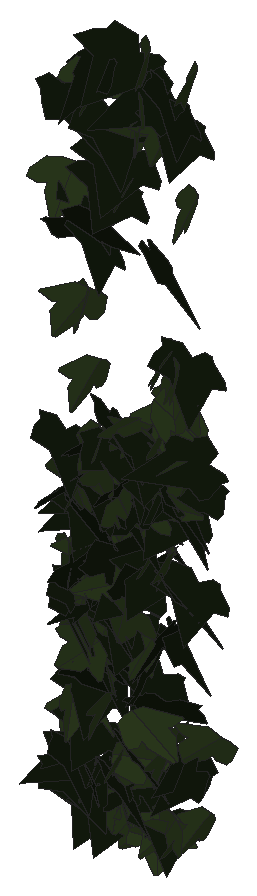
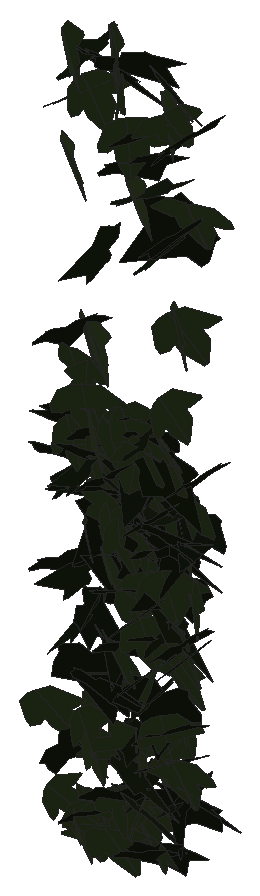
# SketchUp Ruby script. Lengths in inches.
U = 1.inch
M = Sketchup.active_model
def pt(a) = Geom::Point3d.new(a.map { |v| v * U })
def face(e, loops, mat)
  f = e.add_face(loops[0].map { |a| pt(a) })
  loops[1..].each { |l| e.add_face(l.map { |a| pt(a) }).erase! }
  f.material = f.back_material = mat if mat
  f
end
# faces: each face lists its corners as indices into pts; further lists are holes
def faces(e, pts, list, mat = nil) = list.each { |f| face(e, (f[0].is_a?(Array) ? f : [f]).map { |l| l.map { |i| pts[i] } }, mat) }
# xy, xz, yz: faces in a plane at the given z, y or x. An outline is a flat list of corners, or four numbers for a rectangle; further outlines are holes
def ring(l) = l.size == 4 ? [[l[0], l[1]], [l[2], l[1]], [l[2], l[3]], [l[0], l[3]]] : l.each_slice(2).to_a
def flat(e, list, mat, &to3) = list.each { |f| face(e, (f[0].is_a?(Array) ? f : [f]).map { |l| ring(l).map { |u, v| to3.(u, v) } }, mat) }
def xy(e, z, list, mat = nil) = flat(e, list, mat) { |x, y| [x, y, z] }
def xz(e, y, list, mat = nil) = flat(e, list, mat) { |x, z| [x, y, z] }
def yz(e, x, list, mat = nil) = flat(e, list, mat) { |y, z| [x, y, z] }
def lines(e, pts, list) = list.each { |a, b| e.add_line(pt(pts[a]), pt(pts[b])) }
# prism: a flat outline (further loops are holes) pulled along v
def prism(e, loops, v, mat = nil)
  f = face(e, loops, mat); d = Geom::Vector3d.new(v.map { |x| x * U })
  f.pushpull(f.normal.samedirection?(d) ? d.length : -d.length)
end
def box(e, o, s, mat = nil) = prism(e, [[o, [o[0] + s[0], o[1], o[2]], [o[0] + s[0], o[1] + s[1], o[2]], [o[0], o[1] + s[1], o[2]]]], [0, 0, s[2]], mat)
def at(x, y, z, deg = 0) = Geom::Transformation.translation(pt([x, y, z])) * Geom::Transformation.rotation(ORIGIN, Z_AXIS, deg.degrees)
def axes(o, x, y, z) = Geom::Transformation.new([*x, 0, *y, 0, *z, 0, *pt(o).to_a, 1])
def part(name) = M.definitions.add(name)
# library, detail: a bought-in or finely detailed component or shape, given as its bounding box
def library(name, o, s) = part(name).tap { |d| box(d.entities, o, s) }
def detail(e, o, s) = box(e.add_group.entities, o, s)
def put(e, d, t, mat = nil) = e.add_instance(d, t).tap { |i| i.material = mat if mat }
def group(e, t, mat = nil) = e.add_group.tap { |g| g.transformation = t; g.material = mat if mat }.entities
root = M.entities
M.materials.add("1026 AP 7946 SUNNY SIDE UP").color = [254, 231, 186]
M.materials.add("efeu1").color = [18, 25, 13]
M.materials.add("efeu2").color = [43, 57, 29]
c1 = part("ivyleaf_9")
p = [[1.54,2.16,1.25],[1.36,2.04,1.19],[-0.21,0.99,0.68],[-0.71,1.11,0.82],[-0.85,0.86,0.67],[-0.8,0.17,0.21],
  [-0.9,-0.01,0.1],[-0.67,-0.16,-0.02],[-0.08,-0.08,-0.05],[-0.03,-0.6,-0.4],[0.65,-0.88,-0.66],[0.83,-0.6,-0.49],
  [1.29,-0.42,-0.43],[1.8125,-0.07,-0.26],[1.21,0.44,0.15]]
faces(c1.entities,p,[[0,1,2,3,4,5,6,7,8,9,10,11,12,13,14]],"efeu1")
c2 = part("ivyleaf_10")
p = [[0,0.5,-0.03],[-0.0625,2.02,-0.43],[-0.19,2.01,-0.46],[-0.54,1.05,-0.29],[-0.52,0.625,-0.18],[-0.83,0.76,-0.28],
  [-1.16,0.64,-0.33],[-1.15,0.33,-0.24],[-0.77,-0.39,0.02],[-0.3,-0.51,0.16],[0.04,-0.48,0.23],[-0.02,2.01,-0.4375],
  [-0.06,2.01,-0.43],[0.04,-0.49,0.23],[0.67,-0.49,0.14],[1.38,0.36,-0.2],[1.375,0.51,-0.24],[0.81,0.65,-0.19],
  [0.62,0.59,-0.15],[0.6,1.09,-0.28],[0.5,1.23,-0.31]]
faces(c2.entities,p,[[0,1,2,3,4,5,6,7,8,9,10],[11,12,0,13,14,15,16,17,18,19,20]],"efeu2")
put(root,c1,axes([116.8,212.3,272.73],[0.11017,0.25618,0.13801],[0.05388,0.128,-0.27286],[-0.45031,0.07799,0.00112]),"1026 AP 7946 SUNNY SIDE UP")
put(root,c2,axes([116.82,212.65,272.72],[0.1225,-0.25561,-0.10606],[-0.04117,0.09812,-0.27469],[0.43048,0.08212,0.00391]),"1026 AP 7946 SUNNY SIDE UP")
put(root,c2,axes([116.8,212.47,271.73],[0.22805,-0.21005,-0.12772],[-0.0326,0.13175,-0.25665],[0.38118,0.13693,0.05446]),"1026 AP 7946 SUNNY SIDE UP")
put(root,c2,axes([116.78,212.79,269.29],[0.40893,0.02168,-0.05836],[-0.09133,0.01527,-0.268],[-0.02811,0.26575,0.02173]),"1026 AP 7946 SUNNY SIDE UP")
put(root,c1,axes([117,212.56,268.79],[-0.4104,0.01771,0.02308],[-0.03858,-0.03545,-0.26702],[-0.02274,-0.25954,0.0365]),"1026 AP 7946 SUNNY SIDE UP")
put(root,c1,axes([116.67,212.59,273.41],[-0.02183,-0.28584,0.04041],[-0.0034,-0.04079,-0.29506],[0.45401,-0.01405,-0.00027]),"1026 AP 7946 SUNNY SIDE UP")
put(root,c2,axes([116.76,212.55,277.26],[0.46657,0.05221,-0.03464],[-0.04289,-0.03946,-0.30864],[-0.088,0.29604,-0.03322]),"1026 AP 7946 SUNNY SIDE UP")
put(root,c1,axes([116.67,212.79,270.91],[0.04526,-0.27109,0.02421],[-0.00744,-0.02567,-0.28089],[0.42801,0.02822,-0.00744]),"1026 AP 7946 SUNNY SIDE UP")
put(root,c2,axes([117.09,212.45,270.9],[-0.21954,0.13083,0.21379],[-0.33102,0.05714,-0.18334],[-0.19614,-0.24288,0.07012]),"1026 AP 7946 SUNNY SIDE UP")
put(root,c1,axes([116.64,212.62,278.45],[0.13508,-0.28326,-0.10763],[-0.00728,0.10571,-0.30325],[0.4738,0.08238,0.02603]),"1026 AP 7946 SUNNY SIDE UP")
put(root,c1,axes([116.72,212.81,271.12],[-0.00572,-0.27971,-0.00531],[-0.00211,0.00359,-0.28815],[0.43984,-0.00362,-0.00145]),"1026 AP 7946 SUNNY SIDE UP")
put(root,c2,axes([116.86,212.55,272.92],[-0.43647,0.05098,-0.02968],[0.03875,-0.02645,-0.29006],[-0.08377,-0.27784,0.02048]),"1026 AP 7946 SUNNY SIDE UP")
put(root,c2,axes([117,212.54,275.53],[-0.23482,-0.21491,0.16004],[-0.06896,-0.15721,-0.26631],[0.41237,-0.14867,0.0466]),"1026 AP 7946 SUNNY SIDE UP")
put(root,c2,axes([116.85,212.55,269.61],[0.06416,0.22553,-0.1485],[-0.02434,-0.14488,-0.23678],[-0.42126,0.04272,-0.00894]),"1026 AP 7946 SUNNY SIDE UP")
put(root,c1,axes([117.13,212.78,272.46],[-0.43068,0.05972,0.00846],[-0.01834,-0.01663,-0.28825],[-0.09292,-0.27351,0.0177]),"1026 AP 7946 SUNNY SIDE UP")
put(root,c2,axes([116.92,212.84,278.66],[0.26812,0.21109,-0.15435],[-0.11163,-0.13588,-0.27902],[-0.39255,0.18281,-0.02608]),"1026 AP 7946 SUNNY SIDE UP")
put(root,c2,axes([116.98,212.84,269.85],[-0.24545,-0.21557,0.05732],[0.01059,-0.07394,-0.27018],[0.3504,-0.14877,0.04831]),"1026 AP 7946 SUNNY SIDE UP")
put(root,c1,axes([117.0625,212.48,268.72],[0.17257,-0.01247,-0.25671],[-0.38054,0.06053,-0.11261],[0.0949,0.2654,0.01526]),"1026 AP 7946 SUNNY SIDE UP")
put(root,c1,axes([116.78,212.87,277.03],[0.05506,-0.29844,-0.03977],[-0.00588,0.03672,-0.30934],[0.47281,0.03521,0.00078]),"1026 AP 7946 SUNNY SIDE UP")
put(root,c2,axes([117.01,212.73,274.4],[-0.10231,-0.25018,0.14867],[0.02311,-0.15203,-0.263],[0.45468,-0.04857,0.04682]),"1026 AP 7946 SUNNY SIDE UP")
put(root,c1,axes([117.21,212.875,272.64],[-0.42962,0.00079,0.06113],[-0.09186,-0.05248,-0.27674],[0.01631,-0.27462,0.0514]),"1026 AP 7946 SUNNY SIDE UP")
put(root,c1,axes([117.16,212.625,273.46],[-0.09378,0.24669,-0.12343],[0.00527,-0.12338,-0.26109],[-0.43217,-0.05504,0.0236]),"1026 AP 7946 SUNNY SIDE UP")
put(root,c2,axes([117.07,212.69,271.83],[-0.31265,-0.18899,0.06939],[-0.00898,-0.0909,-0.27627],[0.31592,-0.18962,0.06081]),"1026 AP 7946 SUNNY SIDE UP")
put(root,c1,axes([116.83,212.58,268.75],[0.03707,-0.26163,0.10666],[0.04398,-0.10269,-0.27063],[0.44111,0.03223,0.01802]),"1026 AP 7946 SUNNY SIDE UP")
put(root,c1,axes([116.97,212.85,269.76],[-0.16699,-0.2477,0.03137],[0.01363,-0.03826,-0.27687],[0.39246,-0.10407,0.02296]),"1026 AP 7946 SUNNY SIDE UP")
put(root,c1,axes([117.05,212.87,268.1],[-0.32164,-0.15592,-0.03351],[0.05965,0.00226,-0.26407],[0.24295,-0.20697,0.02047]),"1026 AP 7946 SUNNY SIDE UP")
put(root,c1,axes([117.22,212.49,271.24],[-0.26058,0.22191,-0.0552],[0.03561,-0.05146,-0.28534],[-0.35767,-0.1668,0.01181]),"1026 AP 7946 SUNNY SIDE UP")
put(root,c2,axes([117.05,212.48,275.55],[0.20251,-0.25936,-0.06125],[-0.0095,0.06156,-0.29713],[0.41777,0.12712,0.02294]),"1026 AP 7946 SUNNY SIDE UP")
put(root,c1,axes([117.03,212.82,272.38],[-0.2351,-0.23696,0.04936],[0.01399,-0.06324,-0.28596],[0.3803,-0.14416,0.04103]),"1026 AP 7946 SUNNY SIDE UP")
put(root,c2,axes([117.11,212.61,278.68],[0.12774,-0.27589,-0.1203],[-0.02856,0.11461,-0.29527],[0.46925,0.08208,0.01478]),"1026 AP 7946 SUNNY SIDE UP")
put(root,c1,axes([117.03,212.48,272.4],[0.36695,-0.02613,-0.15604],[-0.24041,-0.01388,-0.24053],[0.0225,0.27779,-0.02505]),"1026 AP 7946 SUNNY SIDE UP")
put(root,c2,axes([117.19,212.41,270.54],[0.34925,-0.1127,-0.14779],[-0.20274,0.0615,-0.25621],[0.20182,0.2568,-0.00163]),"1026 AP 7946 SUNNY SIDE UP")
put(root,c1,axes([117.02,212.3,271.74],[-0.04223,0.0915,-0.28021],[-0.09387,0.26596,0.09962],[0.44216,0.0652,-0.00562]),"1026 AP 7946 SUNNY SIDE UP")
put(root,c1,axes([116.91,212.49,268.64],[-0.18108,-0.1399,-0.21192],[0.23475,0.14137,-0.18504],[0.31162,-0.18779,0.01625]),"1026 AP 7946 SUNNY SIDE UP")
put(root,c1,axes([117.08,212.75,269.22],[-0.21601,-0.21098,0.08886],[0.00548,-0.10397,-0.25339],[0.35908,-0.12533,0.05732]),"1026 AP 7946 SUNNY SIDE UP")
put(root,c2,axes([117.25,212.56,273.3125],[-0.40818,0.10329,0.06144],[-0.11627,-0.02903,-0.28274],[-0.14657,-0.26464,0.05319]),"1026 AP 7946 SUNNY SIDE UP")
put(root,c1,axes([117.19,212.58,270.12],[0.25985,0.19688,-0.09219],[-0.0912,-0.06961,-0.26521],[-0.32835,0.17514,0.0007]),"1026 AP 7946 SUNNY SIDE UP")
put(root,c1,axes([117.25,212.58,279.03],[-0.39991,0.06316,-0.17445],[0.23544,-0.09116,-0.26668],[-0.16009,-0.29184,0.04359]),"1026 AP 7946 SUNNY SIDE UP")
put(root,c2,axes([117.42,212.32,273.3],[-0.29849,0.12307,0.18766],[-0.29347,0.03526,-0.22557],[-0.18093,-0.26023,0.05629]),"1026 AP 7946 SUNNY SIDE UP")
put(root,c2,axes([117.16,212.81,268.125],[0.33533,-0.13624,0.05662],[0.05222,-0.05106,-0.25977],[0.22549,0.21443,-0.02405]),"1026 AP 7946 SUNNY SIDE UP")
put(root,c2,axes([117.23,212.47,273.59],[0.26522,-0.23496,0.01684],[-0.00468,-0.02387,-0.29763],[0.37046,0.16791,-0.01582]),"1026 AP 7946 SUNNY SIDE UP")
put(root,c2,axes([117.19,212.51,268.81],[0.22188,-0.21426,0.09681],[0.06469,-0.08675,-0.26449],[0.36293,0.14645,-0.01204]),"1026 AP 7946 SUNNY SIDE UP")
put(root,c1,axes([117.125,212.87,272.82],[-0.04178,-0.277,0.03984],[-0.00314,-0.04024,-0.2869],[0.44012,-0.02658,0.00174]),"1026 AP 7946 SUNNY SIDE UP")
put(root,c1,axes([117.01,212.23,276.81],[0.39791,0.13337,0.10034],[0.16177,0.01035,-0.29218],[-0.20223,0.27069,-0.0363]),"1026 AP 7946 SUNNY SIDE UP")
put(root,c1,axes([117.22,212.94,267.99],[-0.25959,-0.19786,0.00631],[0.05887,-0.04046,-0.25967],[0.30571,-0.16022,0.05536]),"1026 AP 7946 SUNNY SIDE UP")
put(root,c2,axes([117.34,212.78,271.1],[-0.2361,-0.22099,0.06918],[-0.00979,-0.07766,-0.273],[0.36361,-0.14558,0.03756]),"1026 AP 7946 SUNNY SIDE UP")
put(root,c1,axes([117.08,212.68,271.14],[0.22434,-0.23329,0.03435],[0.00825,-0.03737,-0.28151],[0.37076,0.14199,-0.01452]),"1026 AP 7946 SUNNY SIDE UP")
put(root,c1,axes([117.18,212.74,272.6875],[-0.11571,-0.22496,0.16508],[0.10928,-0.17677,-0.22206],[0.42153,-0.01593,0.10288]),"1026 AP 7946 SUNNY SIDE UP")
put(root,c1,axes([117.19,212.61,276.5],[-0.01404,-0.27398,0.14416],[0.00617,-0.14164,-0.28312],[0.48482,-0.00613,0.00778]),"1026 AP 7946 SUNNY SIDE UP")
put(root,c1,axes([117.18,212.83,270.14],[0.09163,-0.26439,0.04178],[-0.00087,-0.04316,-0.27898],[0.42095,0.05746,-0.00967]),"1026 AP 7946 SUNNY SIDE UP")
put(root,c1,axes([117.2,212.8125,270.56],[0.12247,-0.25643,-0.05969],[-0.01453,0.0562,-0.27565],[0.41261,0.07809,0.00801]),"1026 AP 7946 SUNNY SIDE UP")
put(root,c2,axes([117.39,212.59,270.26],[-0.14504,0.25264,0.05003],[-0.05675,0.03684,-0.27602],[-0.4001,-0.09681,0.02102]),"1026 AP 7946 SUNNY SIDE UP")
put(root,c2,axes([117.41,212.53,269.78],[0.07033,-0.27276,0.07869],[0.01143,-0.07777,-0.28516],[0.44591,0.04501,-0.0051]),"1026 AP 7946 SUNNY SIDE UP")
put(root,c1,axes([117.65,212.64,268.52],[-0.25066,0.19666,0.06124],[-0.10786,0.01851,-0.25732],[-0.30397,-0.16874,0.0408]),"1026 AP 7946 SUNNY SIDE UP")
put(root,c2,axes([117.49,212.67,268.3125],[-0.35282,-0.12344,0.03908],[-0.00733,-0.0696,-0.25737],[0.20326,-0.21679,0.05856]),"1026 AP 7946 SUNNY SIDE UP")
put(root,c1,axes([117.64,212.8,269.06],[-0.3005,0.18011,-0.06084],[0.0202,-0.07278,-0.26731],[-0.29787,-0.18664,0.04325]),"1026 AP 7946 SUNNY SIDE UP")
put(root,c1,axes([117.35,212.69,278.26],[-0.07402,-0.30667,-0.03236],[0.01616,0.02843,-0.31941],[0.48419,-0.04783,0.00571]),"1026 AP 7946 SUNNY SIDE UP")
put(root,c1,axes([117.34,212.87,271.33],[0.02515,-0.27496,0.03402],[-0.00033,-0.03465,-0.28394],[0.43576,0.01584,-0.00218]),"1026 AP 7946 SUNNY SIDE UP")
put(root,c2,axes([117.51,212.78,273.54],[-0.43159,0.0527,-0.03429],[0.02665,-0.08286,-0.27709],[-0.09459,-0.26382,0.07841]),"1026 AP 7946 SUNNY SIDE UP")
put(root,c2,axes([117.73,212.4375,271.65],[0.28994,-0.00765,-0.23025],[-0.35091,0.01149,-0.19005],[0.02159,0.28949,0.00315]),"1026 AP 7946 SUNNY SIDE UP")
put(root,c2,axes([117.5,212.66,268.47],[-0.17259,0.23702,0.00899],[-0.02354,0.00119,-0.26875],[-0.37213,-0.11001,0.01283]),"1026 AP 7946 SUNNY SIDE UP")
put(root,c1,axes([117.45,212.68,277.27],[-0.22448,-0.23913,0.14654],[0.04556,-0.17316,-0.2684],[0.43623,-0.10497,0.10344]),"1026 AP 7946 SUNNY SIDE UP")
put(root,c2,axes([117.55,212.85,271.6],[-0.03323,-0.19133,0.20766],[0.04858,-0.20359,-0.19589],[0.43553,0.00811,0.03769]),"1026 AP 7946 SUNNY SIDE UP")
put(root,c2,axes([117.58,212.68,277.3],[0.1895,-0.28166,0.01123],[-0.00812,-0.0158,-0.31551],[0.44325,0.12013,-0.01058]),"1026 AP 7946 SUNNY SIDE UP")
put(root,c1,axes([117.67,212.78,279.23],[-0.40158,-0.18069,0.04766],[-0.04003,-0.04569,-0.32174],[0.29095,-0.25568,0.02152]),"1026 AP 7946 SUNNY SIDE UP")
put(root,c1,axes([117.56,212.73,277.75],[-0.2516,-0.26179,0.03389],[-0.00022,-0.04012,-0.3156],[0.41518,-0.15867,0.02037]),"1026 AP 7946 SUNNY SIDE UP")
put(root,c2,axes([117.85,212.61,273.68],[0.2128,0.00459,-0.26474],[-0.40235,0.03003,-0.13808],[0.03844,0.28891,0.02027]),"1026 AP 7946 SUNNY SIDE UP")
put(root,c2,axes([117.63,212.83,272.47],[-0.15794,-0.26154,0.04765],[0.00614,-0.05248,-0.28803],[0.418,-0.09805,0.02224]),"1026 AP 7946 SUNNY SIDE UP")
put(root,c2,axes([117.56,212.79,272.4375],[0.38297,-0.15084,0.01125],[0.00065,-0.02166,-0.29466],[0.23791,0.24288,-0.01731]),"1026 AP 7946 SUNNY SIDE UP")
put(root,c1,axes([117.56,212.89,270.88],[-0.22073,-0.23496,0.02092],[0.02385,-0.03412,-0.28042],[0.37025,-0.13788,0.03054]),"1026 AP 7946 SUNNY SIDE UP")
put(root,c2,axes([117.63,212.73,278.18],[-0.26818,-0.26187,0.00463],[0.04474,-0.02562,-0.31973],[0.40943,-0.16873,0.03797]),"1026 AP 7946 SUNNY SIDE UP")
put(root,c1,axes([117.36,212.67,273.86],[0.16679,-0.26056,0.08481],[0.03667,-0.08094,-0.29016],[0.42882,0.10827,-0.00817]),"1026 AP 7946 SUNNY SIDE UP")
put(root,c2,axes([117.67,212.73,268.55],[-0.32616,-0.15938,0.01059],[0.01489,-0.03056,-0.26789],[0.25079,-0.20547,0.02968]),"1026 AP 7946 SUNNY SIDE UP")
put(root,c2,axes([117.88,212.83,267.97],[-0.29057,-0.10201,0.14897],[-0.18505,-0.08641,-0.21737],[0.2088,-0.21854,0.01466]),"1026 AP 7946 SUNNY SIDE UP")
put(root,c2,axes([117.74,212.36,269.18],[0.06625,-0.23832,-0.13864],[-0.0237,0.13256,-0.24844],[0.42865,0.04416,0.00769]),"1026 AP 7946 SUNNY SIDE UP")
put(root,c1,axes([117.77,212.78,271.51],[-0.34523,-0.15368,0.07448],[-0.00533,-0.11546,-0.26096],[0.26759,-0.20057,0.0909]),"1026 AP 7946 SUNNY SIDE UP")
put(root,c1,axes([117.54,212.35,271.8],[-0.04158,-0.06093,0.28913],[0.38102,0.14718,0.05723],[-0.24337,0.24083,0.0402]),"1026 AP 7946 SUNNY SIDE UP")
put(root,c1,axes([117.74,212.33,273.08],[0.09691,0.25946,0.10374],[0.05687,0.09328,-0.27387],[-0.43308,0.07031,-0.01275]),"1026 AP 7946 SUNNY SIDE UP")
put(root,c2,axes([117.77,212.58,273.9],[-0.08709,-0.28103,0.0589],[-0.01427,-0.05811,-0.29541],[0.45122,-0.05608,0.00202]),"1026 AP 7946 SUNNY SIDE UP")
put(root,c1,axes([117.48,212.58,268.66],[0.19268,-0.23169,0.08001],[0.04506,-0.07414,-0.27029],[0.38225,0.12553,-0.00847]),"1026 AP 7946 SUNNY SIDE UP")
put(root,c2,axes([117.87,212.36,271.33],[-0.42807,0.0593,0.09415],[-0.15002,-0.01289,-0.2853],[-0.08178,-0.28677,0.03054]),"1026 AP 7946 SUNNY SIDE UP")
put(root,c1,axes([117.58,212.49,273.65],[-0.04822,-0.245,-0.17388],[0.07132,0.16243,-0.25253],[0.46108,-0.05075,0.02088]),"1026 AP 7946 SUNNY SIDE UP")
put(root,c2,axes([117.98,212.63,273.57],[-0.40174,-0.00026,0.1502],[-0.22543,-0.05301,-0.25923],[0.04166,-0.28935,0.04561]),"1026 AP 7946 SUNNY SIDE UP")
put(root,c1,axes([117.71,212.86,268.65],[-0.18637,-0.21642,-0.09178],[0.08362,0.07094,-0.25349],[0.35763,-0.12937,0.01144]),"1026 AP 7946 SUNNY SIDE UP")
put(root,c2,axes([117.75,212.36,272.85],[-0.03334,-0.25659,-0.11694],[0.13263,0.1013,-0.25482],[0.4198,-0.05238,0.07122]),"1026 AP 7946 SUNNY SIDE UP")
put(root,c2,axes([117.85,212.72,270.63],[0.33812,-0.18371,-0.03661],[-0.05234,0.0141,-0.29107],[0.28922,0.21732,-0.00987]),"1026 AP 7946 SUNNY SIDE UP")
put(root,c2,axes([117.89,212.73,273.83],[-0.03839,-0.24747,0.15139],[-0.00959,-0.14841,-0.25694],[0.45359,-0.02408,0.00738]),"1026 AP 7946 SUNNY SIDE UP")
put(root,c1,axes([117.62,212.67,272.58],[0.21053,-0.25127,0.01916],[-0.00538,-0.02448,-0.29308],[0.39632,0.13315,-0.01415]),"1026 AP 7946 SUNNY SIDE UP")
put(root,c2,axes([117.88,212.74,272.5625],[-0.02876,-0.28063,0.00044],[0.01133,-0.00249,-0.28963],[0.44112,-0.01823,0.00747]),"1026 AP 7946 SUNNY SIDE UP")
put(root,c2,axes([117.92,212.79,271.97],[0.13392,-0.27185,-0.00405],[-0.00177,0.00215,-0.29347],[0.42747,0.08518,0.00006]),"1026 AP 7946 SUNNY SIDE UP")
put(root,c1,axes([117.68,212.56,269.24],[0.28451,-0.19341,0.01059],[-0.00314,-0.01743,-0.2726],[0.30462,0.18046,-0.01271]),"1026 AP 7946 SUNNY SIDE UP")
put(root,c2,axes([117.95,212.62,279.35],[0.17345,-0.2795,-0.09131],[0.0115,0.09563,-0.3062],[0.46016,0.10296,0.04207]),"1026 AP 7946 SUNNY SIDE UP")
put(root,c1,axes([117.8125,212.44,271.5],[0.00492,-0.03166,0.29153],[0.32047,0.19815,0.02166],[-0.3131,0.20231,0.02676]),"1026 AP 7946 SUNNY SIDE UP")
put(root,c2,axes([117.94,212.52,278.68],[-0.19566,0.25686,-0.12068],[-0.04158,-0.13956,-0.2836],[-0.44291,-0.10037,0.07994]),"1026 AP 7946 SUNNY SIDE UP")
put(root,c1,axes([118.05,212.33,272.71],[-0.32041,0.19749,-0.07499],[-0.07634,0.05609,0.29259],[0.32267,0.20938,-0.00524]),"1026 AP 7946 SUNNY SIDE UP")
put(root,c1,axes([117.8,212.68,272.53],[0.43823,-0.01095,-0.06201],[-0.09459,0.00059,-0.28733],[0.01703,0.28511,-0.00011]),"1026 AP 7946 SUNNY SIDE UP")
put(root,c1,axes([117.89,212.86,273.16],[-0.12872,-0.26542,0.05592],[-0.00599,-0.05715,-0.28617],[0.42642,-0.08092,0.01286]),"1026 AP 7946 SUNNY SIDE UP")
put(root,c1,axes([118.01,212.875,270.17],[-0.38635,-0.07466,-0.09578],[0.15462,-0.00811,-0.26225],[0.10513,-0.26243,0.0337]),"1026 AP 7946 SUNNY SIDE UP")
put(root,c2,axes([117.82,212.43,269.11],[0.04543,0.03988,0.28195],[0.17332,0.25047,-0.04817],[-0.39848,0.11349,0.0112]),"1026 AP 7946 SUNNY SIDE UP")
put(root,c2,axes([117.86,212.8,272.66],[-0.32116,0.10359,-0.17303],[0.19606,-0.12069,-0.23278],[-0.24152,-0.23571,0.04114]),"1026 AP 7946 SUNNY SIDE UP")
put(root,c2,axes([117.89,212.61,273.29],[0.4208,0.04999,0.08582],[0.11154,0.06509,-0.27555],[-0.10382,0.27253,0.05181]),"1026 AP 7946 SUNNY SIDE UP")
put(root,c1,axes([118.05,212.72,271.9],[-0.24389,-0.23154,0.0477],[-0.01463,-0.05092,-0.28664],[0.3714,-0.15405,0.02003]),"1026 AP 7946 SUNNY SIDE UP")
put(root,c1,axes([118.31,212.52,278.91],[-0.48067,0.05418,0.01254],[-0.02961,-0.03886,-0.31718],[-0.08203,-0.30344,0.041]),"1026 AP 7946 SUNNY SIDE UP")
put(root,c1,axes([118.25,212.27,270.5],[-0.15878,0.04506,-0.29923],[-0.34734,0.19139,0.11072],[0.30551,0.24101,-0.02963]),"1026 AP 7946 SUNNY SIDE UP")
put(root,c2,axes([118.02,212.78,267.95],[0.3214,0.16327,-0.00521],[0.0135,-0.02031,-0.26874],[-0.25655,0.20348,-0.02067]),"1026 AP 7946 SUNNY SIDE UP")
put(root,c2,axes([118.14,212.77,273.81],[0.09183,-0.28716,-0.0173],[0.02792,0.01904,-0.30099],[0.4513,0.05726,0.02214]),"1026 AP 7946 SUNNY SIDE UP")
put(root,c2,axes([118.21,212.81,268.09],[-0.12469,-0.14676,0.20437],[-0.01975,-0.20654,-0.16311],[0.38857,-0.05759,0.05729]),"1026 AP 7946 SUNNY SIDE UP")
put(root,c1,axes([118.11,212.7,273.72],[-0.19258,-0.26505,0.01525],[0.00634,-0.01981,-0.30066],[0.41751,-0.12196,0.0116]),"1026 AP 7946 SUNNY SIDE UP")
put(root,c2,axes([118.2,212.75,269.16],[0.01989,-0.26791,0.02179],[0.00623,-0.02251,-0.27642],[0.42272,0.01294,0.00305]),"1026 AP 7946 SUNNY SIDE UP")
put(root,c1,axes([117.95,212.79,276.375],[0.30839,-0.23795,-0.03672],[-0.054,0.01607,-0.31714],[0.37414,0.19845,-0.01551]),"1026 AP 7946 SUNNY SIDE UP")
put(root,c2,axes([118.23,212.68,275.01],[0.1219,-0.28341,-0.05247],[-0.04042,0.04405,-0.30214],[0.45053,0.08064,-0.01291]),"1026 AP 7946 SUNNY SIDE UP")
put(root,c2,axes([118.27,212.7,268.11],[-0.29759,-0.17242,0.02094],[-0.00503,-0.02803,-0.26323],[0.27313,-0.18838,0.01796]),"1026 AP 7946 SUNNY SIDE UP")
put(root,c1,axes([118.15,212.83,268.21],[-0.12512,-0.24295,-0.01592],[0.03042,0.00845,-0.26282],[0.38145,-0.08037,0.01574]),"1026 AP 7946 SUNNY SIDE UP")
put(root,c2,axes([118.3,212.8,269.47],[-0.0391,-0.26933,0.03368],[0.01162,-0.03502,-0.27864],[0.42674,-0.02372,0.01067]),"1026 AP 7946 SUNNY SIDE UP")
put(root,c2,axes([118.29,212.66,272.08],[0.11658,-0.26852,-0.00962],[0.01416,0.01058,-0.28667],[0.42217,0.0738,0.01227]),"1026 AP 7946 SUNNY SIDE UP")
put(root,c2,axes([118.32,212.78,274.14],[-0.36416,-0.16555,0.05235],[0.03579,-0.1146,-0.27337],[0.27038,-0.2078,0.1067]),"1026 AP 7946 SUNNY SIDE UP")
put(root,c2,axes([118.35,212.63,278.52],[-0.17126,-0.27512,0.10005],[-0.0024,-0.10477,-0.30327],[0.45958,-0.10307,0.0357]),"1026 AP 7946 SUNNY SIDE UP")
put(root,c1,axes([118.33,212.69,271.05],[-0.16915,0.09863,-0.24044],[0.20382,-0.19714,-0.14818],[-0.34327,-0.16565,0.03049]),"1026 AP 7946 SUNNY SIDE UP")
put(root,c2,axes([118.35,212.61,268.24],[0.31578,-0.14284,-0.10806],[-0.09261,0.09445,-0.25006],[0.26202,0.20553,0.04185]),"1026 AP 7946 SUNNY SIDE UP")
put(root,c2,axes([118.38,212.76,268],[0.08137,-0.26162,-0.0159],[-0.0091,0.01307,-0.27464],[0.41185,0.05198,-0.00293]),"1026 AP 7946 SUNNY SIDE UP")
put(root,c1,axes([118.46,212.4,270.15],[0.18446,0.18138,-0.16415],[-0.16469,-0.12264,-0.22255],[-0.34322,0.15633,0.01856]),"1026 AP 7946 SUNNY SIDE UP")
put(root,c2,axes([118.15,212.3,269.81],[0.22477,0.18263,0.15978],[0.16612,0.11271,-0.23798],[-0.33698,0.17738,-0.01074]),"1026 AP 7946 SUNNY SIDE UP")
put(root,c1,axes([118.39,212.83,272.8],[-0.34222,-0.18379,0.02484],[0.04955,-0.07485,-0.28292],[0.28745,-0.20591,0.07835]),"1026 AP 7946 SUNNY SIDE UP")
put(root,c2,axes([118.05,212.51,272.9],[-0.12366,0.01563,0.30023],[0.45403,0.04744,0.07795],[-0.06579,0.29802,-0.02636]),"1026 AP 7946 SUNNY SIDE UP")
put(root,c2,axes([118.36,212.51,274.38],[0.00608,0.23852,0.18328],[0.01791,0.17631,-0.24462],[-0.46627,0.00988,-0.00701]),"1026 AP 7946 SUNNY SIDE UP")
put(root,c2,axes([118.47,212.52,274.95],[0.25283,-0.24226,-0.06027],[-0.02478,0.05797,-0.29859],[0.39059,0.16049,0.02007]),"1026 AP 7946 SUNNY SIDE UP")
put(root,c1,axes([118.29,212.73,270.96],[0.25496,-0.19967,-0.1024],[-0.10253,0.07362,-0.26452],[0.33457,0.17472,-0.00303]),"1026 AP 7946 SUNNY SIDE UP")
put(root,c1,axes([118.24,212.76,273.14],[0.23873,-0.24674,0.00335],[-0.01587,-0.01166,-0.29814],[0.38772,0.15145,-0.01426]),"1026 AP 7946 SUNNY SIDE UP")
put(root,c1,axes([118.24,212.82,271.65],[0.27328,-0.22051,0.02359],[0.0395,-0.01091,-0.289],[0.34656,0.17513,0.01434]),"1026 AP 7946 SUNNY SIDE UP")
put(root,c1,axes([118.42,212.79,278.47],[-0.14221,-0.27413,0.11546],[0.03201,-0.12424,-0.29281],[0.46551,-0.0752,0.05541]),"1026 AP 7946 SUNNY SIDE UP")
put(root,c1,axes([118.55,212.94,269.1],[0.01343,-0.0512,-0.26673],[0.13752,-0.24355,0.05122],[-0.39107,-0.0874,0.00885]),"1026 AP 7946 SUNNY SIDE UP")
put(root,c2,axes([118.57,212.6,274.51],[0.39248,-0.14209,-0.07038],[-0.07294,0.05451,-0.29455],[0.23637,0.25276,0.02597]),"1026 AP 7946 SUNNY SIDE UP")
put(root,c2,axes([118.57,212.77,279.17],[0.14422,-0.30081,0.01365],[0.03631,-0.00857,-0.3234],[0.47218,0.09253,0.0207]),"1026 AP 7946 SUNNY SIDE UP")
put(root,c1,axes([118.71,212.83,273.28],[-0.41118,-0.11402,0.03967],[-0.01809,-0.0695,-0.28803],[0.1887,-0.25512,0.05883]),"1026 AP 7946 SUNNY SIDE UP")
put(root,c2,axes([118.61,212.66,273.52],[-0.12749,-0.2758,0.03548],[0.02123,-0.04136,-0.29532],[0.43683,-0.07848,0.02471]),"1026 AP 7946 SUNNY SIDE UP")
put(root,c1,axes([118.4375,212.6,278.875],[-0.00211,-0.26615,0.17963],[0.02678,-0.17569,-0.27478],[0.5009,0.00827,0.01545]),"1026 AP 7946 SUNNY SIDE UP")
put(root,c1,axes([118.72,212.65,269.12],[-0.38172,0.05967,-0.09189],[0.12948,-0.0392,-0.25715],[-0.1089,-0.25576,0.01636]),"1026 AP 7946 SUNNY SIDE UP")
put(root,c1,axes([118.89,212.67,273.67],[-0.39543,-0.03601,0.14411],[-0.19582,-0.08902,-0.2544],[0.11569,-0.27376,0.06197]),"1026 AP 7946 SUNNY SIDE UP")
put(root,c1,axes([118.44,212.71,272.9375],[0.14152,-0.25897,0.06763],[0.02792,-0.06487,-0.28279],[0.41974,0.09163,-0.00399]),"1026 AP 7946 SUNNY SIDE UP")
put(root,c1,axes([118.57,212.79,275.04],[-0.10742,-0.28875,0.0072],[-0.00063,-0.00878,-0.30572],[0.45423,-0.0683,0.00128]),"1026 AP 7946 SUNNY SIDE UP")
put(root,c1,axes([118.62,212.85,271.74],[-0.16912,-0.25742,0.02611],[0.00033,-0.02911,-0.28734],[0.40696,-0.10695,0.01109]),"1026 AP 7946 SUNNY SIDE UP")
put(root,c2,axes([118.69,212.61,277.46],[0.25055,-0.26084,-0.00112],[-0.01029,-0.00446,-0.3148],[0.41001,0.15928,-0.00722]),"1026 AP 7946 SUNNY SIDE UP")
put(root,c2,axes([118.9,212.83,269.55],[-0.28247,-0.09925,0.17279],[-0.20925,-0.10524,-0.21089],[0.22493,-0.22253,0.02081]),"1026 AP 7946 SUNNY SIDE UP")
put(root,c2,axes([118.71,212.85,268.32],[-0.0526,-0.17767,0.18795],[0.02907,-0.18622,-0.18341],[0.40051,-0.00982,0.03799]),"1026 AP 7946 SUNNY SIDE UP")
